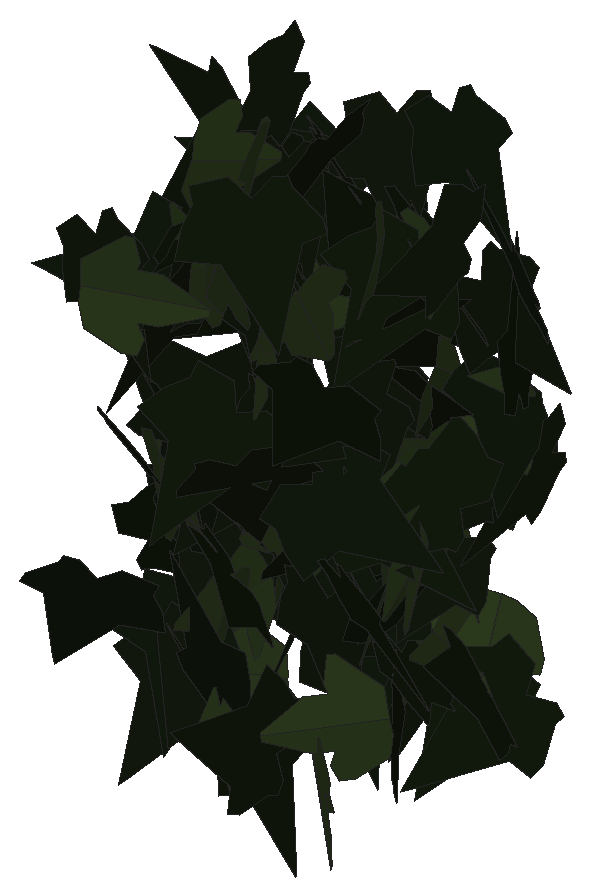
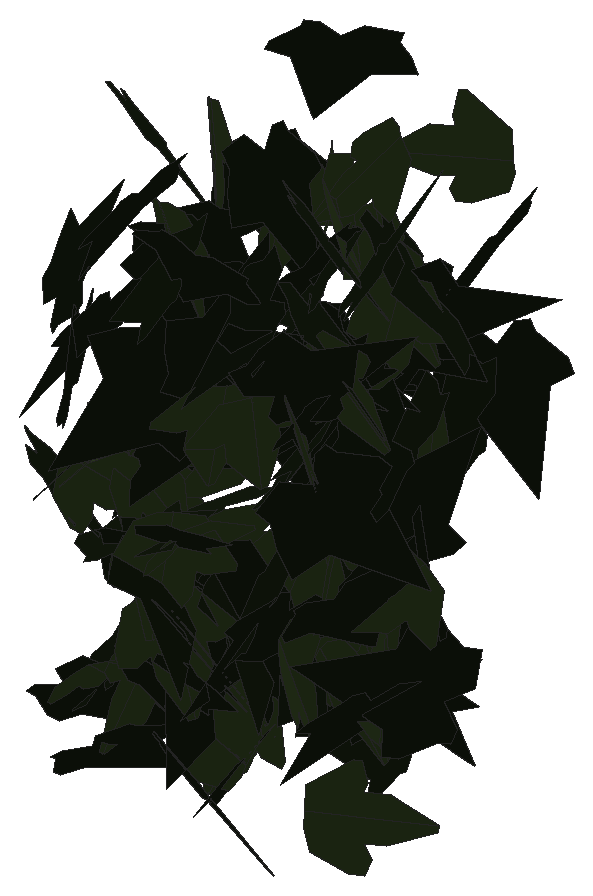
# SketchUp Ruby script. Lengths in inches.
U = 1.inch
M = Sketchup.active_model
def pt(a) = Geom::Point3d.new(a.map { |v| v * U })
def face(e, loops, mat)
  f = e.add_face(loops[0].map { |a| pt(a) })
  loops[1..].each { |l| e.add_face(l.map { |a| pt(a) }).erase! }
  f.material = f.back_material = mat if mat
  f
end
# faces: each face lists its corners as indices into pts; further lists are holes
def faces(e, pts, list, mat = nil) = list.each { |f| face(e, (f[0].is_a?(Array) ? f : [f]).map { |l| l.map { |i| pts[i] } }, mat) }
# xy, xz, yz: faces in a plane at the given z, y or x. An outline is a flat list of corners, or four numbers for a rectangle; further outlines are holes
def ring(l) = l.size == 4 ? [[l[0], l[1]], [l[2], l[1]], [l[2], l[3]], [l[0], l[3]]] : l.each_slice(2).to_a
def flat(e, list, mat, &to3) = list.each { |f| face(e, (f[0].is_a?(Array) ? f : [f]).map { |l| ring(l).map { |u, v| to3.(u, v) } }, mat) }
def xy(e, z, list, mat = nil) = flat(e, list, mat) { |x, y| [x, y, z] }
def xz(e, y, list, mat = nil) = flat(e, list, mat) { |x, z| [x, y, z] }
def yz(e, x, list, mat = nil) = flat(e, list, mat) { |y, z| [x, y, z] }
def lines(e, pts, list) = list.each { |a, b| e.add_line(pt(pts[a]), pt(pts[b])) }
# prism: a flat outline (further loops are holes) pulled along v
def prism(e, loops, v, mat = nil)
  f = face(e, loops, mat); d = Geom::Vector3d.new(v.map { |x| x * U })
  f.pushpull(f.normal.samedirection?(d) ? d.length : -d.length)
end
def box(e, o, s, mat = nil) = prism(e, [[o, [o[0] + s[0], o[1], o[2]], [o[0] + s[0], o[1] + s[1], o[2]], [o[0], o[1] + s[1], o[2]]]], [0, 0, s[2]], mat)
def at(x, y, z, deg = 0) = Geom::Transformation.translation(pt([x, y, z])) * Geom::Transformation.rotation(ORIGIN, Z_AXIS, deg.degrees)
def axes(o, x, y, z) = Geom::Transformation.new([*x, 0, *y, 0, *z, 0, *pt(o).to_a, 1])
def part(name) = M.definitions.add(name)
# library, detail: a bought-in or finely detailed component or shape, given as its bounding box
def library(name, o, s) = part(name).tap { |d| box(d.entities, o, s) }
def detail(e, o, s) = box(e.add_group.entities, o, s)
def put(e, d, t, mat = nil) = e.add_instance(d, t).tap { |i| i.material = mat if mat }
def group(e, t, mat = nil) = e.add_group.tap { |g| g.transformation = t; g.material = mat if mat }.entities
root = M.entities
M.materials.add("efeu1").color = [18, 25, 13]
M.materials.add("efeu2").color = [43, 57, 29]
c1 = part("ivyleaf_9")
p = [[1.54,2.16,1.25],[1.36,2.04,1.19],[-0.21,0.99,0.68],[-0.71,1.11,0.82],[-0.85,0.86,0.67],[-0.8,0.17,0.21],
  [-0.9,-0.01,0.1],[-0.67,-0.16,-0.02],[-0.08,-0.08,-0.05],[-0.03,-0.6,-0.4],[0.65,-0.88,-0.66],[0.83,-0.6,-0.49],
  [1.29,-0.42,-0.43],[1.8125,-0.07,-0.26],[1.21,0.44,0.15]]
faces(c1.entities,p,[[0,1,2,3,4,5,6,7,8,9,10,11,12,13,14]],"efeu1")
c2 = part("ivyleaf_10")
p = [[0,0.5,-0.03],[-0.0625,2.02,-0.43],[-0.19,2.01,-0.46],[-0.54,1.05,-0.29],[-0.52,0.625,-0.18],[-0.83,0.76,-0.28],
  [-1.16,0.64,-0.33],[-1.15,0.33,-0.24],[-0.77,-0.39,0.02],[-0.3,-0.51,0.16],[0.04,-0.48,0.23],[-0.02,2.01,-0.4375],
  [-0.06,2.01,-0.43],[0.04,-0.49,0.23],[0.67,-0.49,0.14],[1.38,0.36,-0.2],[1.375,0.51,-0.24],[0.81,0.65,-0.19],
  [0.62,0.59,-0.15],[0.6,1.09,-0.28],[0.5,1.23,-0.31]]
faces(c2.entities,p,[[0,1,2,3,4,5,6,7,8,9,10],[11,12,0,13,14,15,16,17,18,19,20]],"efeu2")
put(root,c1,axes([44.53,220.43,243.42],[0.1694,0.03257,0.4693],[0.4582,0.10158,-0.17245],[-0.10657,0.48849,0.00456]))
put(root,c1,axes([45.1875,221.48,245.96],[-0.05822,0.20449,-0.45254],[-0.24433,-0.40847,-0.15315],[-0.43233,0.20331,0.14749]))
put(root,c1,axes([45.17,220.4375,245.01],[0.1678,0.06244,0.46685],[-0.46621,-0.04851,0.17406],[0.06703,-0.49371,0.04194]))
put(root,c1,axes([45.11,220.95,247.91],[0.14121,-0.47666,0.05348],[-0.01497,0.05135,0.49713],[-0.47941,-0.142,0.00023]))
put(root,c2,axes([45.36,221.18,247.12],[-0.3295,0.03281,0.37464],[-0.36535,-0.14604,-0.30853],[0.08918,-0.47707,0.12021]))
put(root,c1,axes([45.18,219.61,247.2],[-0.34508,0.32016,-0.16858],[-0.12398,0.11424,0.47072],[0.33993,0.36667,0.00054]))
put(root,c1,axes([45.14,220.08,244.03],[0.29926,-0.13848,0.37585],[-0.15419,0.39319,0.26764],[-0.36969,-0.27609,0.19263]))
put(root,c1,axes([44.81,220.87,246.34],[0.49033,-0.09268,0.03145],[0.03062,-0.00737,-0.49901],[0.09296,0.49128,-0.00155]))
put(root,c2,axes([44.92,220.46,244.63],[-0.3699,-0.05699,-0.33155],[0.33602,-0.03883,-0.36821],[0.01622,-0.49522,0.06703]))
put(root,c1,axes([45.48,219.67,246.9375],[-0.21728,-0.05287,0.44721],[-0.43408,-0.10755,-0.22362],[0.11984,-0.48542,0.00084]))
put(root,c1,axes([44.93,221.01,243.49],[0.1547,-0.38179,-0.28338],[0.0388,0.30715,-0.39263],[0.47388,0.09949,0.12465]))
put(root,c1,axes([45.48,221.67,247],[-0.11642,0.05501,0.48313],[-0.47016,-0.13949,-0.09742],[0.12406,-0.47699,0.08421]))
put(root,c2,axes([45.47,220.9,242],[-0.01875,0.00056,0.49965],[-0.34061,-0.36583,-0.01237],[0.36556,-0.34083,0.0141]))
put(root,c1,axes([45.1,218.84,247.61],[0.22295,-0.42748,-0.1325],[-0.06738,0.11428,-0.48208],[0.44244,0.23281,-0.00665]))
put(root,c2,axes([45.29,220.1,247.37],[-0.15479,-0.42434,-0.21442],[0.09133,0.19476,-0.45136],[0.46658,-0.1789,0.01722]))
put(root,c1,axes([45.25,221.09,244.55],[-0.17369,-0.46862,0.015],[-0.00445,-0.01434,-0.49977],[0.46884,-0.17375,0.00081]))
put(root,c2,axes([45.19,220.56,243],[-0.00338,-0.29036,-0.40704],[0.12865,-0.39385,0.27988],[-0.48315,-0.10284,0.07737]))
put(root,c1,axes([45.36,220.85,244.47],[-0.15327,-0.39003,0.27274],[-0.08144,-0.26081,-0.41874],[0.46891,-0.17278,0.01642]))
put(root,c1,axes([45.28,220.03,243.01],[-0.08501,-0.48989,0.05279],[-0.00933,-0.05196,-0.49721],[0.49263,-0.08551,-0.00031]))
put(root,c1,axes([45.21,221.21,246.86],[0.06944,-0.48785,-0.08474],[-0.01739,0.08311,-0.49274],[0.49485,0.07138,-0.00543]))
put(root,c2,axes([45.36,221.57,246.7],[0.33629,-0.36213,0.07595],[0.0529,-0.05453,-0.49419],[0.36621,0.34042,0.00164]))
put(root,c1,axes([45.74,220.86,247.45],[-0.32011,0.37132,0.09822],[-0.07764,0.06267,-0.48994],[-0.37617,-0.32892,0.01754]))
put(root,c1,axes([45.74,219.7,247.8],[-0.37298,0.32851,-0.05451],[0.03581,-0.04181,-0.49696],[-0.33107,-0.37461,0.00766]))
put(root,c2,axes([45.83,219.53,247.25],[-0.26713,0.06741,0.41725],[-0.41857,0.02629,-0.27222],[-0.05863,-0.49474,0.04238]))
put(root,c1,axes([45.35,220.97,246.63],[0.02231,-0.49799,-0.03885],[-0.00158,0.03882,-0.49849],[0.4995,0.02237,0.00015]))
put(root,c2,axes([45.74,220.46,243.33],[0.30425,-0.17221,-0.35746],[-0.30224,0.19125,-0.34939],[0.25706,0.42868,0.01228]))
put(root,c1,axes([45.6875,221.06,248.66],[-0.45831,0.14086,-0.14183],[0.12574,-0.07262,-0.47845],[-0.15539,-0.47422,0.03114]))
put(root,c1,axes([45.1875,220.1,242.64],[0.33286,-0.33179,0.17064],[0.11755,-0.12377,-0.46996],[0.3541,0.35298,-0.00439]))
put(root,c1,axes([45.63,219.57,246.98],[-0.16802,0.17145,-0.43861],[0.22572,-0.37939,-0.23477],[-0.4133,-0.2769,0.05009]))
put(root,c1,axes([45.36,221.07,246.48],[0.27172,-0.41946,-0.015],[-0.00751,0.01301,-0.49977],[0.41966,0.27182,0.00077]))
put(root,c1,axes([45.73,219.63,242.85],[-0.4598,-0.18701,-0.06011],[0.05437,0.02586,-0.49636],[0.18875,-0.46299,-0.00344]))
put(root,c1,axes([46,221.58,247.15],[-0.41178,-0.05941,0.27732],[-0.27649,-0.02474,-0.41586],[0.06314,-0.49584,-0.01248]))
put(root,c2,axes([45.84,218.97,245.27],[-0.42116,0.19617,0.18478],[-0.17608,0.05922,-0.46421],[-0.20401,-0.45608,0.0192]))
put(root,c1,axes([45.36,218.86,245.52],[0.42373,-0.23781,0.11788],[0.09779,-0.06655,-0.48581],[0.24675,0.43476,-0.00988]))
put(root,c2,axes([45.72,221.2,243.75],[0.21951,-0.43926,0.09417],[0.03907,-0.08575,-0.49104],[0.44754,0.22293,-0.00332]))
put(root,c1,axes([45.5,219.58,245.48],[0.29146,-0.35543,0.19679],[0.12762,-0.14984,-0.45963],[0.3857,0.31815,0.00338]))
put(root,c1,axes([46.29,220.24,246.74],[-0.16436,-0.05144,-0.4694],[-0.42537,-0.1997,0.17082],[-0.20505,0.4555,0.02188]))
put(root,c2,axes([45.8,220.57,244.64],[-0.04329,0.06673,-0.49363],[0.14085,-0.47363,-0.07638],[-0.47779,-0.14567,0.02221]))
put(root,c2,axes([45.92,221.54,246.58],[0.25028,0.42702,-0.07082],[-0.03355,-0.06242,-0.49495],[-0.43155,0.25251,-0.00259]))
put(root,c2,axes([46.25,219.28,247.5],[-0.36903,0.10705,0.31994],[-0.30447,0.09857,-0.38417],[-0.14532,-0.47836,-0.00756]))
put(root,c2,axes([45.92,219.5,248.52],[0.00037,-0.19669,-0.45969],[0.17556,0.43047,-0.18404],[0.46817,-0.16127,0.06938]))
put(root,c2,axes([45.96,220.23,248.36],[0.25675,-0.38443,0.19051],[0.11292,-0.15364,-0.46222],[0.41392,0.28038,0.00792]))
put(root,c1,axes([45.83,221.45,247.77],[0.45445,-0.17364,-0.11542],[-0.10393,0.0513,-0.48638],[0.18075,0.46607,0.01053]))
put(root,c1,axes([45.77,220.62,247.67],[0.25465,-0.42613,0.0597],[0.03905,-0.04619,-0.49633],[0.42852,0.25744,0.00976]))
put(root,c1,axes([45.88,220.8125,247.87],[0.06928,-0.49508,-0.0096],[-0.00209,0.0094,-0.49991],[0.49517,0.06931,-0.00077]))
put(root,c2,axes([46.08,219.58,243.71],[0.03316,-0.48395,0.12121],[0.04707,-0.1179,-0.48361],[0.49667,0.04349,0.03774]))
put(root,c1,axes([46.05,220.89,244.02],[0.19066,-0.21466,-0.40935],[-0.09801,0.41397,-0.26273],[0.45171,0.18043,0.11578]))
put(root,c1,axes([46.49,217.07,245.09],[0.1862,0.30371,-0.35084],[-0.22663,-0.27036,-0.35432],[-0.40493,0.29098,0.03698]))
put(root,c2,axes([45.98,217.86,247.76],[0.0055,0.0157,0.49972],[0.39398,0.30755,-0.014],[-0.30782,0.39392,-0.00899]))
put(root,c1,axes([46.5,219.98,243.03],[-0.0207,0.28242,0.41208],[-0.01125,0.41206,-0.28298],[-0.49944,-0.02099,-0.0107]))
put(root,c1,axes([46.51,218.98,243.05],[0.21718,-0.17916,0.4132],[-0.24701,0.3362,0.27561],[-0.37659,-0.32384,0.05752]))
put(root,c2,axes([46.33,220.31,244.23],[-0.47278,-0.10156,-0.12715],[0.12293,0.03306,-0.48352],[0.10662,-0.48846,-0.00629]))
put(root,c1,axes([46.18,219.63,243.88],[-0.05287,-0.26362,0.42156],[0.15303,-0.41198,-0.23844],[0.47306,0.10381,0.12425]))
put(root,c1,axes([46.51,221.39,246.74],[0.13531,0.21898,0.42865],[-0.3442,-0.26723,0.24518],[0.33647,-0.36144,0.07843]))
put(root,c2,axes([46.42,221.04,242.95],[-0.48507,0.04169,-0.1139],[0.11401,-0.0035,-0.48682],[-0.04138,-0.49825,-0.00611]))
put(root,c2,axes([46.37,221.45,246.49],[0.23975,0.43675,0.04205],[0.02007,0.03695,-0.49823],[-0.43831,0.24058,0.00019]))
put(root,c1,axes([46.56,219.08,246.05],[-0.4034,-0.29541,-0.00199],[0.00153,0.00128,-0.5],[0.29541,-0.4034,-0.00013]))
put(root,c1,axes([46.17,221.14,244.1],[0.19931,-0.38563,0.24812],[0.10909,-0.2229,-0.43407],[0.44539,0.22716,-0.00471]))
put(root,c1,axes([46.6,220.48,244.11],[0.09104,0.48185,-0.09763],[-0.02813,-0.09402,-0.49027],[-0.49084,0.09476,0.00999]))
put(root,c1,axes([46.69,220.6,243.81],[-0.08399,0.46516,0.16302],[-0.04253,0.15791,-0.4725],[-0.49106,-0.09324,0.01304]))
put(root,c1,axes([46.27,221.2,242.51],[0.15505,-0.47535,-0.00043],[-0.00043,0.00031,-0.5],[0.47535,0.15505,-0.00031]))
put(root,c1,axes([46.29,220.32,245.36],[0.05363,-0.45021,0.21079],[0.09486,-0.19885,-0.44884],[0.48798,0.08814,0.06409]))
put(root,c1,axes([46.71,220.34,248.59],[-0.18817,0.4157,-0.20442],[0.08828,-0.18442,-0.45628],[-0.45475,-0.20781,-0.00399]))
put(root,c1,axes([46.1875,219.93,245.05],[0.22878,-0.0378,-0.44298],[0.44099,0.08253,0.22072],[0.05643,-0.49169,0.0711]))
put(root,c2,axes([46.57,219.3,242.8],[0.20585,0.44949,-0.07476],[-0.03061,-0.06821,-0.49438],[-0.45463,0.20811,-0.00057]))
put(root,c1,axes([46.49,221.72,248.17],[-0.24219,-0.28477,-0.33204],[0.35123,0.09964,-0.34163],[0.26074,-0.39872,0.15177]))
put(root,c1,axes([47.05,221.33,242.26],[-0.43422,0.22709,0.09942],[-0.08401,0.05387,-0.48994],[-0.23323,-0.44219,-0.00862]))
put(root,c2,axes([46.42,221.27,242.59],[-0.18142,-0.11836,0.45064],[0.45396,0.06397,0.19956],[-0.1049,0.48156,0.08425]))
put(root,c1,axes([47.08,221.21,243.72],[-0.45196,0.21063,0.03694],[-0.0318,0.01921,-0.49862],[-0.21147,-0.45306,-0.00396]))
put(root,c1,axes([46.8,220.88,243.39],[0.30782,0.39313,-0.02636],[-0.00822,-0.02704,-0.4992],[-0.39393,0.30776,-0.01018]))
put(root,c1,axes([46.59,219.42,242.43],[-0.1819,-0.10017,-0.45484],[0.43686,0.13258,-0.20391],[0.16145,-0.47158,0.03929]))
put(root,c2,axes([47.02,221.49,243.91],[-0.40757,-0.23441,0.1701],[-0.15104,-0.07853,-0.47013],[0.24713,-0.43461,-0.0068]))
put(root,c1,axes([46.95,218.71,245.79],[0.24114,0.41959,-0.12567],[-0.05866,-0.11122,-0.48393],[-0.43406,0.24813,-0.00441]))
put(root,c1,axes([47.2,221.27,244.47],[-0.0727,0.49425,0.02086],[-0.00615,0.02018,-0.49955],[-0.49465,-0.0729,0.00314]))
put(root,c2,axes([47.04,221.4375,244.74],[-0.30598,-0.38687,-0.08189],[0.08494,0.03683,-0.49135],[0.38622,-0.3146,0.04318]))
put(root,c1,axes([47.34,221.39,243.92],[-0.46513,0.17287,0.06144],[-0.0546,0.02943,-0.49614],[-0.17515,-0.46824,-0.0085]))
put(root,c2,axes([46.95,221.3,244.62],[-0.26006,-0.37811,0.19851],[0.21952,-0.31772,-0.31759],[0.36631,-0.07803,0.33126]))
put(root,c1,axes([47.09,221.58,243.37],[-0.4367,-0.17641,-0.16785],[0.16108,0.04919,-0.47078],[0.18262,-0.46525,0.01387]))
put(root,c1,axes([47.2,221.67,244.84],[-0.4279,-0.2581,0.01685],[0.04248,-0.10226,-0.48758],[0.25514,-0.41584,0.10945]))
put(root,c1,axes([47.09,220.63,243.68],[-0.08073,-0.49337,-0.00849],[0.00034,0.00855,-0.49993],[0.49344,-0.08073,-0.00104]))
put(root,c1,axes([47.3,218.79,242.73],[-0.02489,-0.02704,0.49865],[-0.31531,-0.3863,-0.03669],[0.38724,-0.31629,0.00218]))
put(root,c1,axes([47.02,220,243.74],[0.11233,-0.47796,0.09451],[0.04327,-0.08682,-0.4905],[0.48529,0.11838,0.02186]))
put(root,c2,axes([47.38,220.37,243.86],[0.16806,-0.36229,-0.30084],[-0.11482,0.27826,-0.39924],[0.4567,0.20327,0.01033]))
put(root,c2,axes([47.13,218.88,247.28],[-0.06168,0.21484,-0.44726],[0.14747,-0.4224,-0.22324],[-0.47376,-0.15945,-0.01126]))
put(root,c1,axes([47.1,221.32,246.42],[0.39153,0.2495,0.18561],[0.16554,0.08541,-0.46401],[-0.26324,0.4248,-0.01572]))
put(root,c2,axes([47.34,219.18,247.55],[-0.12263,-0.42674,-0.22991],[0.067,0.21995,-0.444],[0.48008,-0.1397,0.00324]))
put(root,c1,axes([47.22,220.73,246.11],[-0.12239,-0.4147,0.25109],[0.02391,-0.26382,-0.42406],[0.4842,-0.09179,0.08441]))
put(root,c1,axes([47.24,220.73,245.95],[0.47979,0.12541,-0.06381],[-0.06137,-0.01756,-0.49591],[-0.12662,0.4837,-0.00145]))
put(root,c1,axes([47.3,220.19,243.375],[0.12791,0.20382,0.43829],[0.23658,0.36896,-0.24062],[-0.42151,0.26893,-0.00205]))
put(root,c1,axes([47.12,221.22,247.5625],[0.34948,-0.35308,0.05652],[0.03671,-0.04318,-0.49678],[0.35569,0.35138,-0.00426]))
put(root,c1,axes([47.26,218.52,248.9],[-0.18351,-0.36594,-0.28708],[0.1766,0.23068,-0.40694],[0.43027,-0.25075,0.04458]))
put(root,c2,axes([47.3,220.12,245.12],[0.01616,-0.18671,0.46355],[0.12515,0.45053,0.1771],[-0.48381,0.1103,0.0613]))
put(root,c1,axes([47.54,220.18,246.16],[-0.16388,-0.30099,0.36407],[-0.17038,-0.32175,-0.3427],[0.44058,-0.23639,0.00289]))
put(root,c1,axes([47.29,221.6,248.51],[0.18364,-0.43238,-0.17125],[-0.03547,0.17056,-0.46867],[0.4637,0.18429,0.03197]))
put(root,c1,axes([47.63,221.2,244.12],[-0.47768,-0.13925,-0.0493],[0.0483,0.01049,-0.49755],[0.1396,-0.4801,0.00343]))
put(root,c1,axes([47.16,220.47,244.64],[0.23789,-0.425,-0.11305],[0.21305,0.22381,-0.39309],[0.38473,0.13886,0.28757]))
put(root,c1,axes([47.76,220.09,242.6875],[0.02226,0.0776,-0.49344],[-0.46456,0.18471,0.00809],[0.18355,0.4581,0.08032]))
put(root,c1,axes([47.4375,220.46,243.22],[0.41364,-0.10531,-0.2604],[-0.19113,0.23416,-0.3983],[0.20584,0.42904,0.15346]))
put(root,c2,axes([47.64,221.16,245.2],[0.01442,-0.43052,0.25386],[-0.00122,-0.254,-0.43068],[0.49979,0.0118,-0.00837]))
put(root,c2,axes([47.66,220.61,247.63],[0.4118,-0.24045,-0.15035],[-0.12098,0.09081,-0.47657],[0.25649,0.42888,0.01661]))
put(root,c1,axes([47.46,221.54,244.59],[-0.26005,-0.37848,0.19782],[0.21951,-0.31713,-0.31819],[0.36632,-0.07864,0.33109]))
put(root,c2,axes([47.68,220.86,246.24],[0.05994,-0.29493,-0.39928],[-0.05139,0.39633,-0.30046],[0.49373,0.07705,0.0172]))
put(root,c2,axes([47.57,221.06,243.09],[-0.08921,-0.36989,-0.32439],[0.11194,0.30577,-0.37944],[0.47907,-0.14032,0.02825]))
put(root,c1,axes([47.64,220.09,246.91],[0.19404,0.44947,0.10163],[0.05034,0.08893,-0.48945],[-0.45805,0.20018,-0.01074]))
put(root,c1,axes([47.73,220.46,247.53],[-0.37378,-0.33087,0.02847],[-0.01791,-0.02271,-0.49916],[0.33161,-0.37418,0.00512]))
put(root,c1,axes([47.68,221.74,242.37],[-0.30769,-0.37983,0.10515],[-0.00462,-0.12992,-0.4828],[0.39409,-0.29808,0.07644]))
put(root,c2,axes([47.78,221.8125,245.45],[-0.08844,-0.29841,0.39132],[0.00662,-0.39827,-0.30222],[0.49207,-0.04828,0.0744]))
put(root,c2,axes([47.81,220.64,244.6],[0.01674,-0.40595,0.29141],[0.03012,-0.29023,-0.40603],[0.49881,0.03115,0.01474]))
put(root,c1,axes([48.2,220.48,245.04],[-0.23417,0.19799,0.39493],[-0.40385,0.08526,-0.2822],[-0.17909,-0.45114,0.11998]))
put(root,c1,axes([47.49,219.25,245.53],[0.12154,-0.18747,-0.44731],[0.1977,0.44024,-0.13079],[0.44288,-0.14508,0.18114]))
put(root,c2,axes([47.93,219.62,248.2],[0.19412,-0.37519,-0.26749],[-0.09118,0.25324,-0.42138],[0.45167,0.21238,0.0299]))
put(root,c2,axes([48.19,219.09,243.25],[-0.14179,0.05962,0.47575],[-0.36632,-0.33357,-0.06737],[0.30936,-0.36766,0.13828]))
put(root,c2,axes([47.77,221.65,243.11],[-0.36572,-0.28231,0.19119],[0.22329,-0.41019,-0.17856],[0.25767,-0.04522,0.4261]))
put(root,c2,axes([47.78,221.625,245.42],[-0.36826,-0.1853,0.28293],[0.22425,-0.44689,-0.0008],[0.25317,0.12631,0.41225]))
put(root,c2,axes([47.8,218.9,242.69],[-0.19965,0.29386,-0.35183],[0.17439,-0.30621,-0.35471],[-0.42395,-0.26435,0.01977]))
put(root,c1,axes([48.19,218.46,247.19],[0.19512,0.20514,-0.41212],[-0.32198,-0.25909,-0.28142],[-0.32902,0.37521,0.03099]))
put(root,c1,axes([47.81,221.8125,245.5625],[-0.00986,-0.46511,0.18323],[0.06202,-0.18299,-0.46116],[0.49604,0.01363,0.0613]))
put(root,c2,axes([48.06,220.09,244.55],[0.29845,-0.37868,-0.1324],[-0.04649,0.13126,-0.48022],[0.39845,0.29896,0.04314]))
put(root,c1,axes([47.88,221.35,246.98],[0.2304,-0.29778,-0.32901],[-0.11842,0.31601,-0.36894],[0.42766,0.24793,0.07509]))
put(root,c1,axes([48.37,221.29,242.61],[-0.41327,-0.23443,0.15573],[-0.13645,-0.07507,-0.47513],[0.24615,-0.43521,-0.00193]))
put(root,c1,axes([48.27,221.375,246.02],[0.01797,-0.2597,0.42689],[0.05629,0.42549,0.25649],[-0.4965,0.03884,0.04453]))
put(root,c1,axes([48.125,221.04,242.71],[0.30702,-0.37236,-0.13073],[0.08963,-0.09551,0.48254],[-0.38433,-0.31973,0.0081]))
put(root,c1,axes([48.39,221.43,247],[0.14799,-0.38862,0.27762],[-0.10344,0.25767,0.41582],[-0.46626,-0.18051,-0.00413]))
put(root,c1,axes([48.47,221.59,245.1875],[-0.43959,0.17504,-0.16163],[0.1295,-0.10919,-0.47043],[-0.19999,-0.45545,0.05066]))
put(root,c1,axes([48.03,219,244.75],[0.38625,-0.31372,0.0489],[0.04111,-0.02694,-0.49758],[0.31483,0.3884,0.00498]))
put(root,c1,axes([48.65,219.99,248.3],[-0.40835,0.27829,0.07623],[-0.06738,0.03648,-0.49409],[-0.28056,-0.4138,0.00771]))
